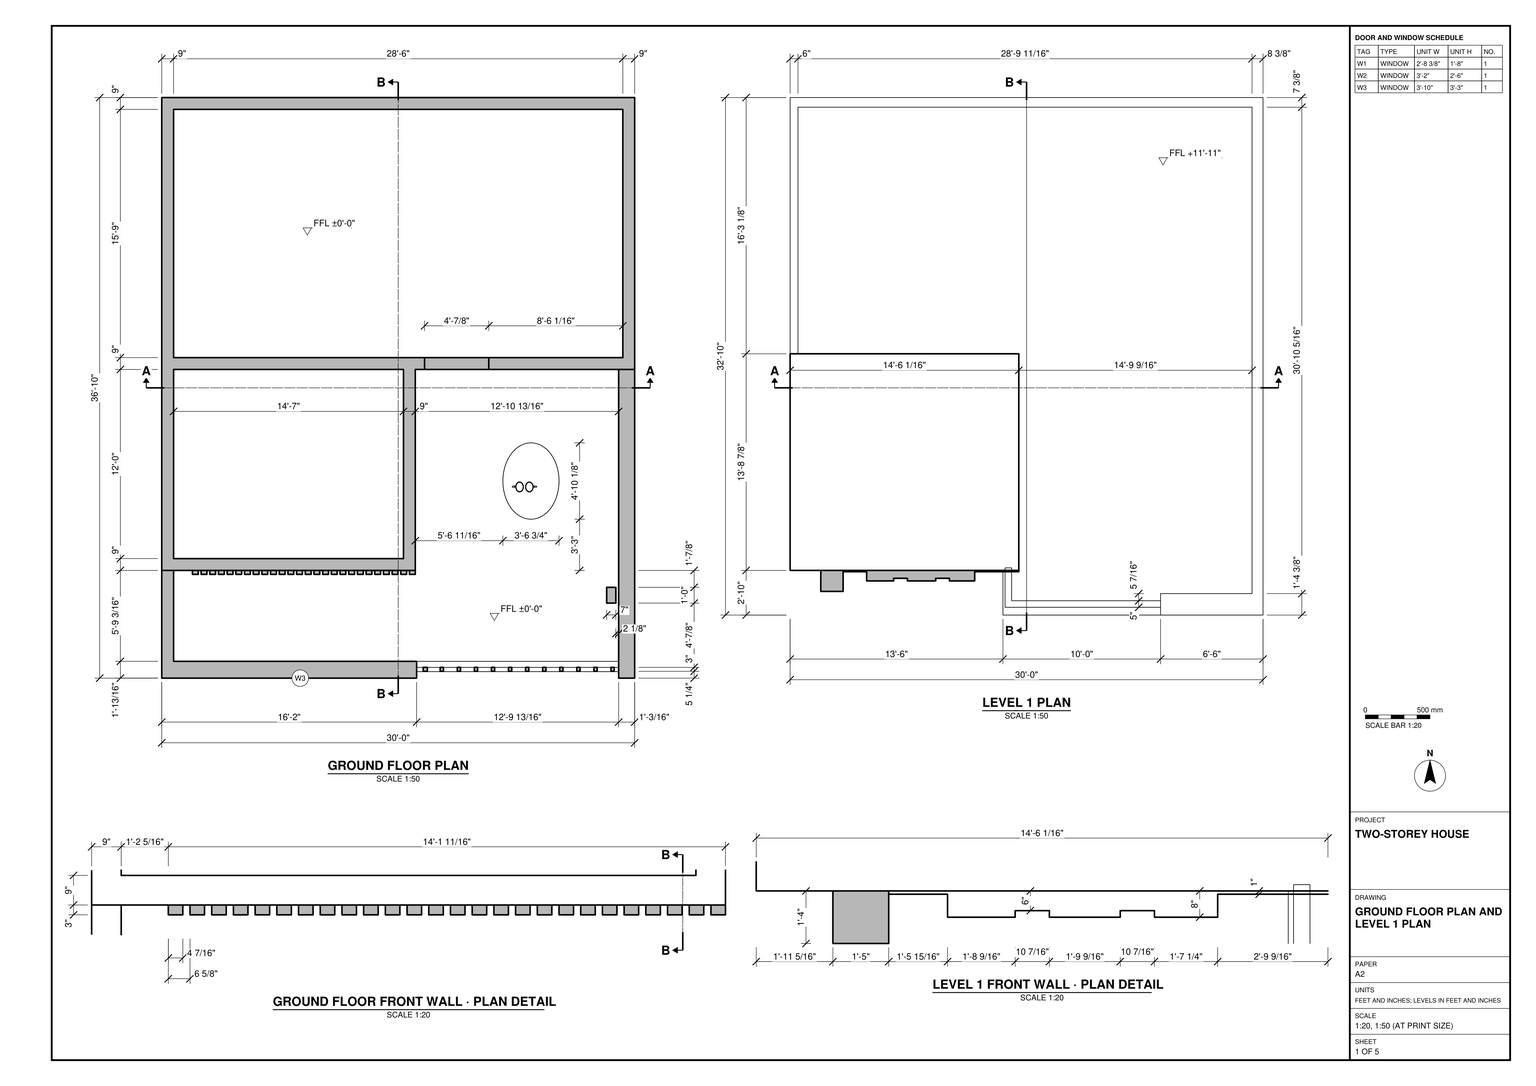
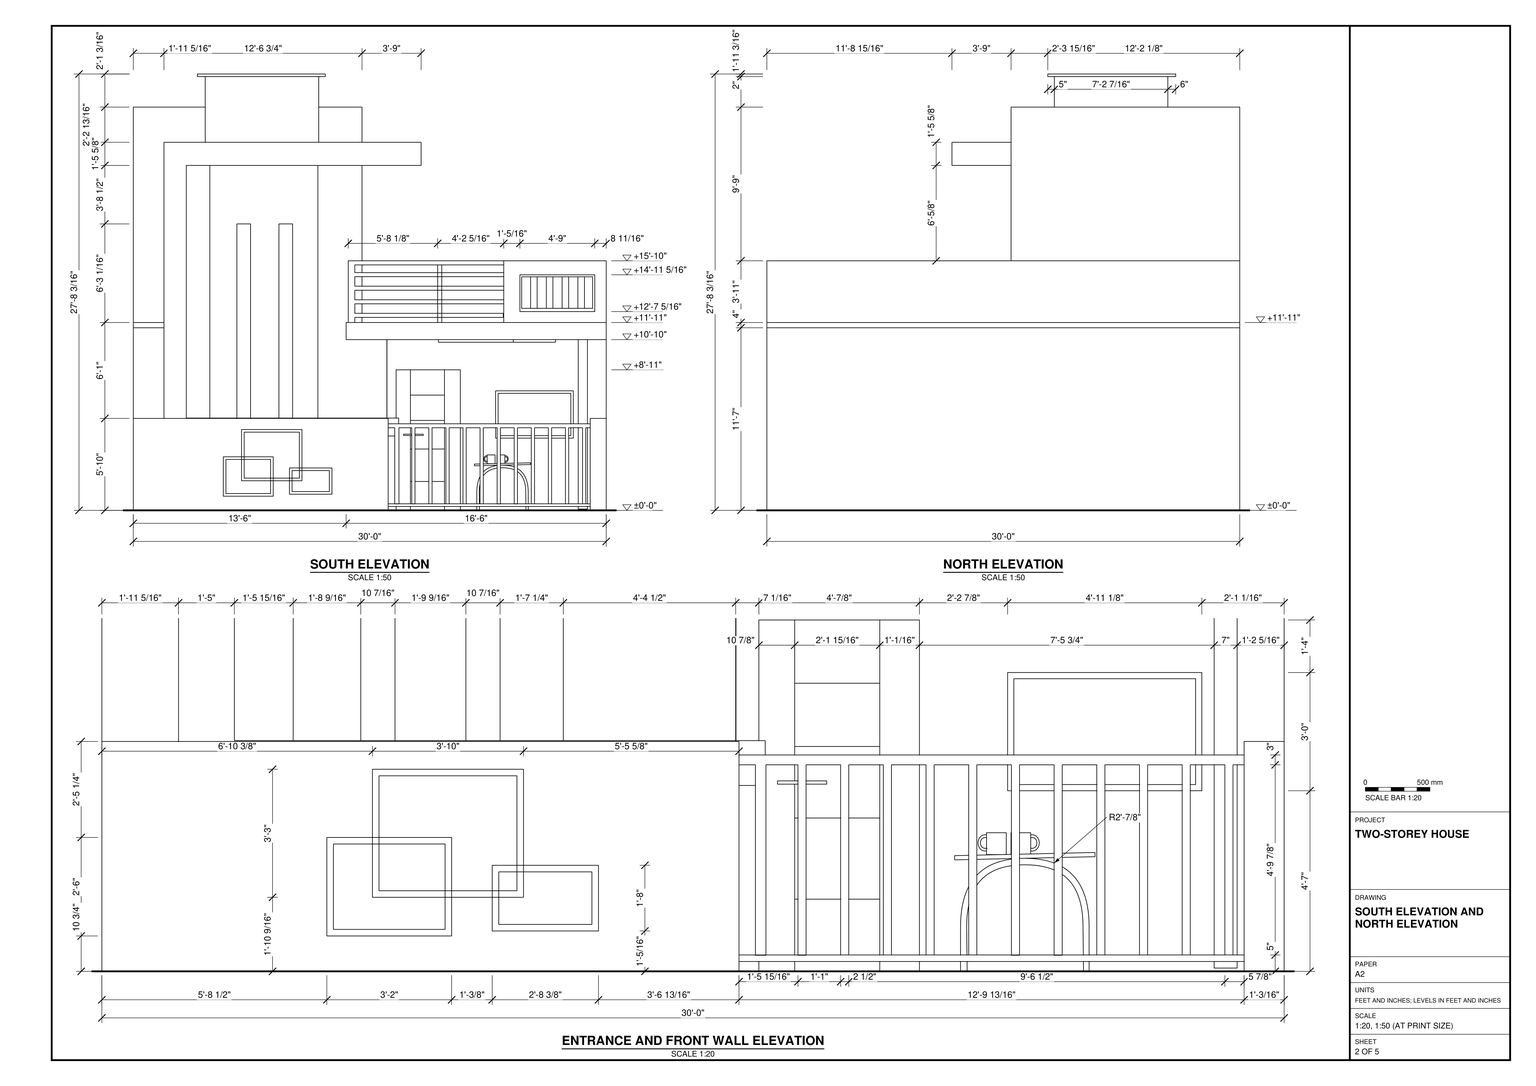
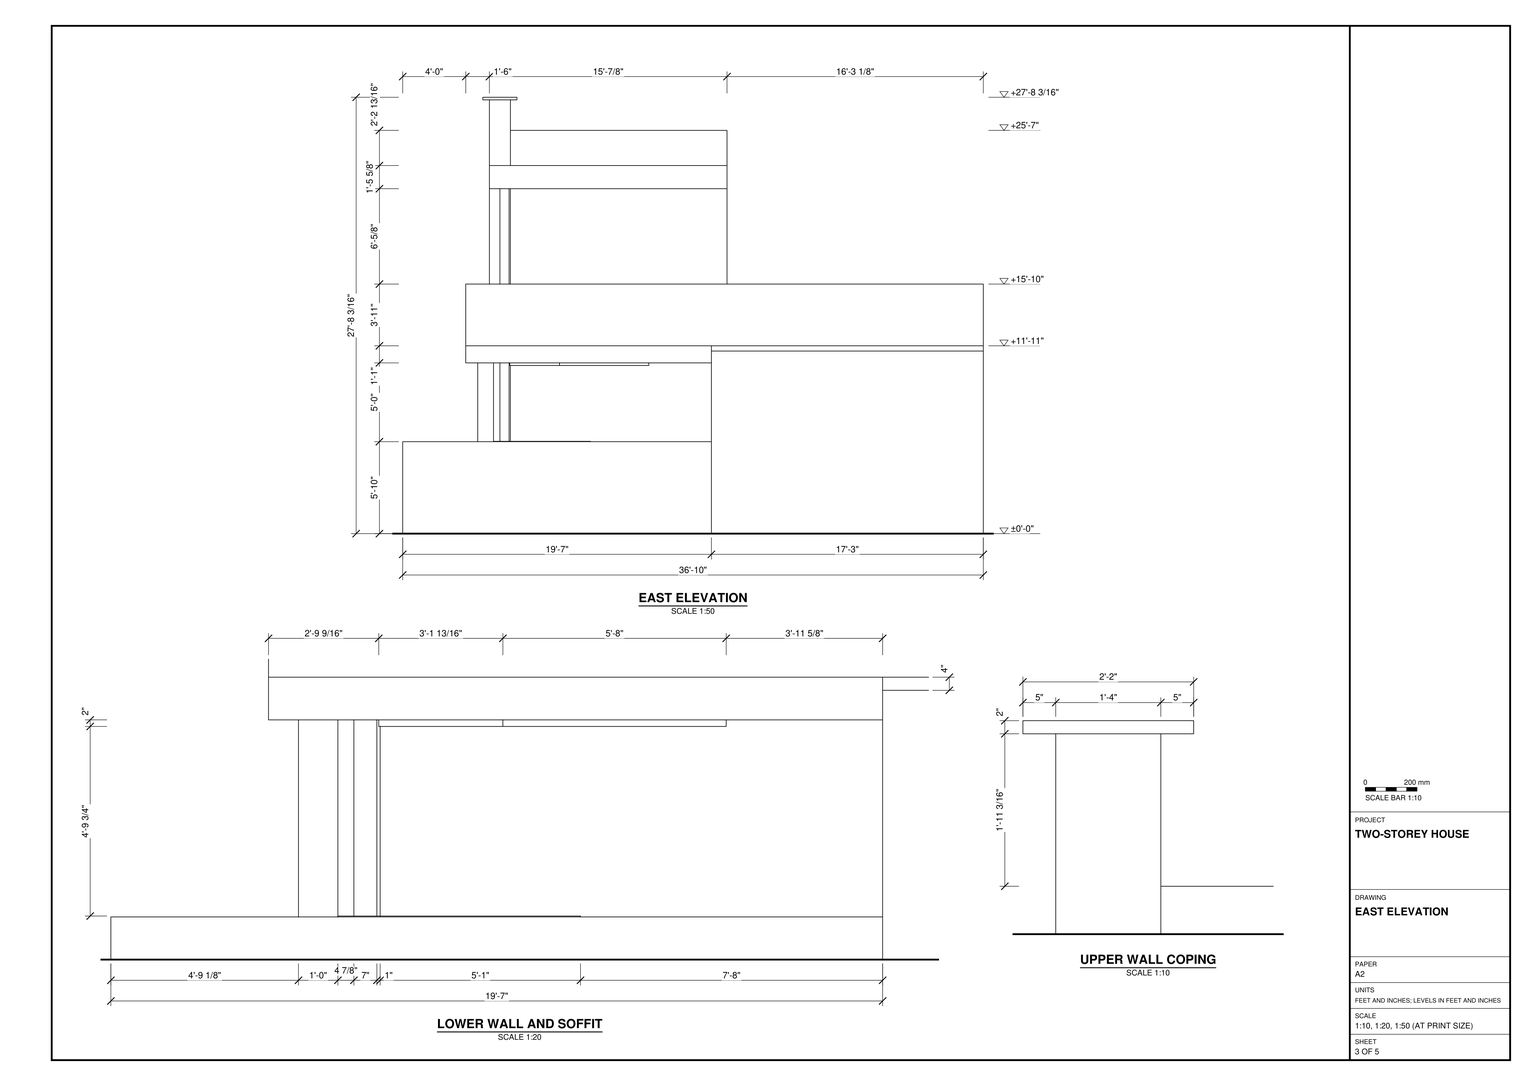
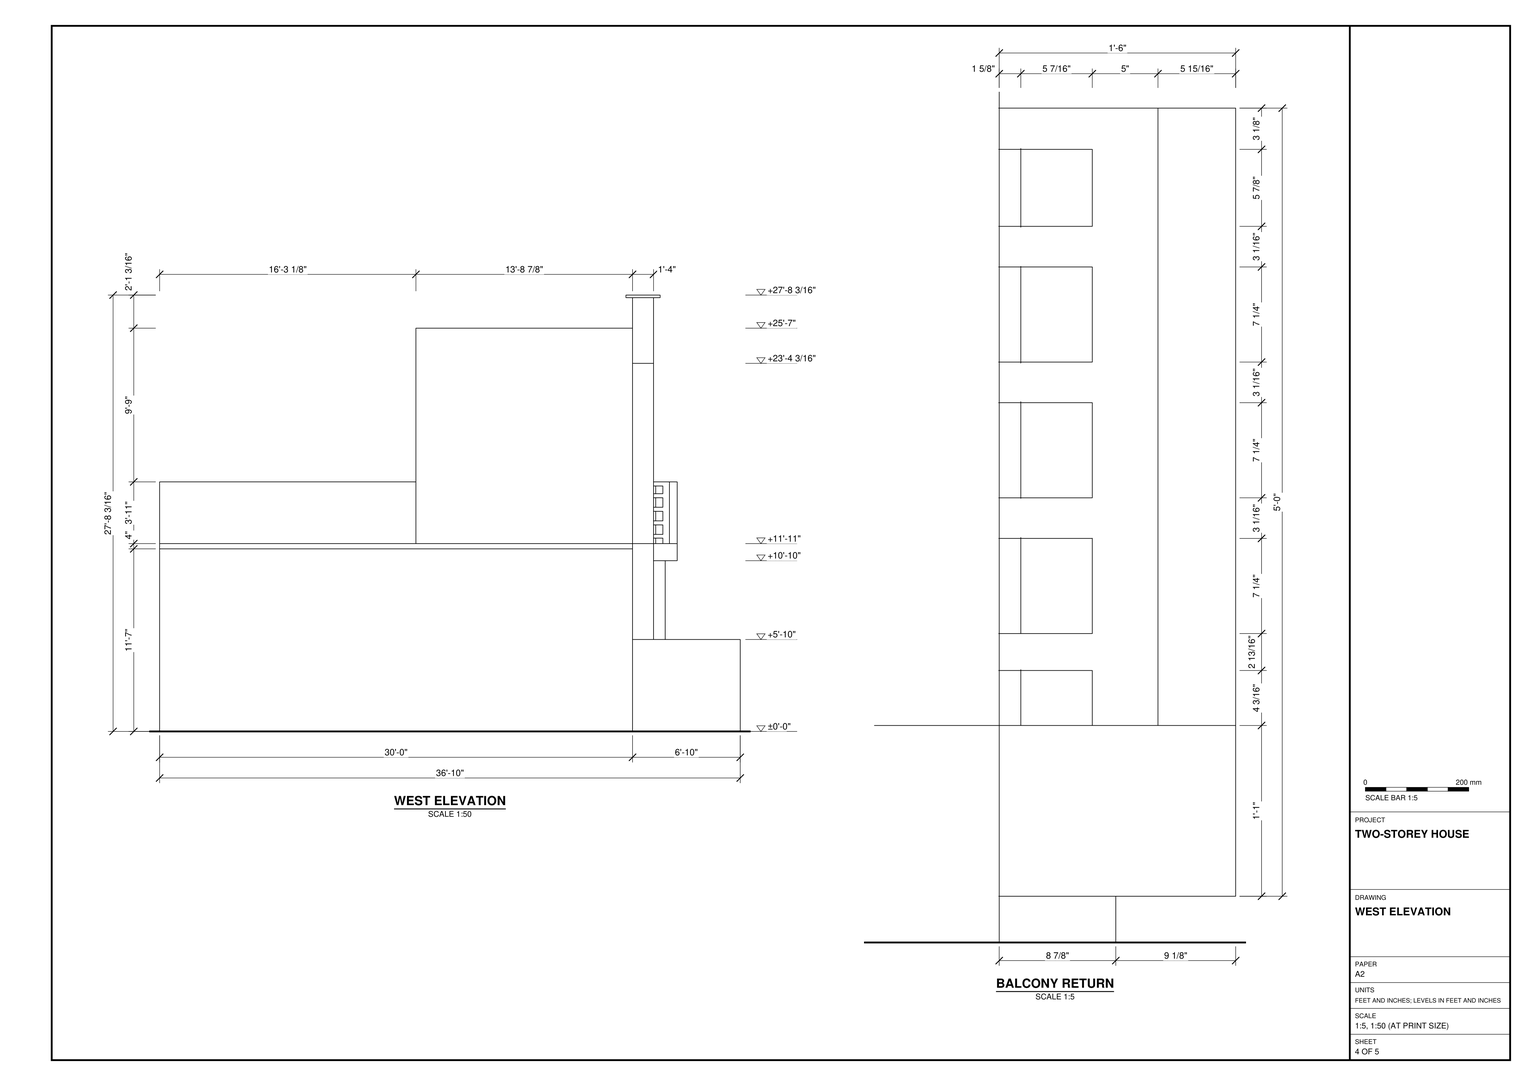
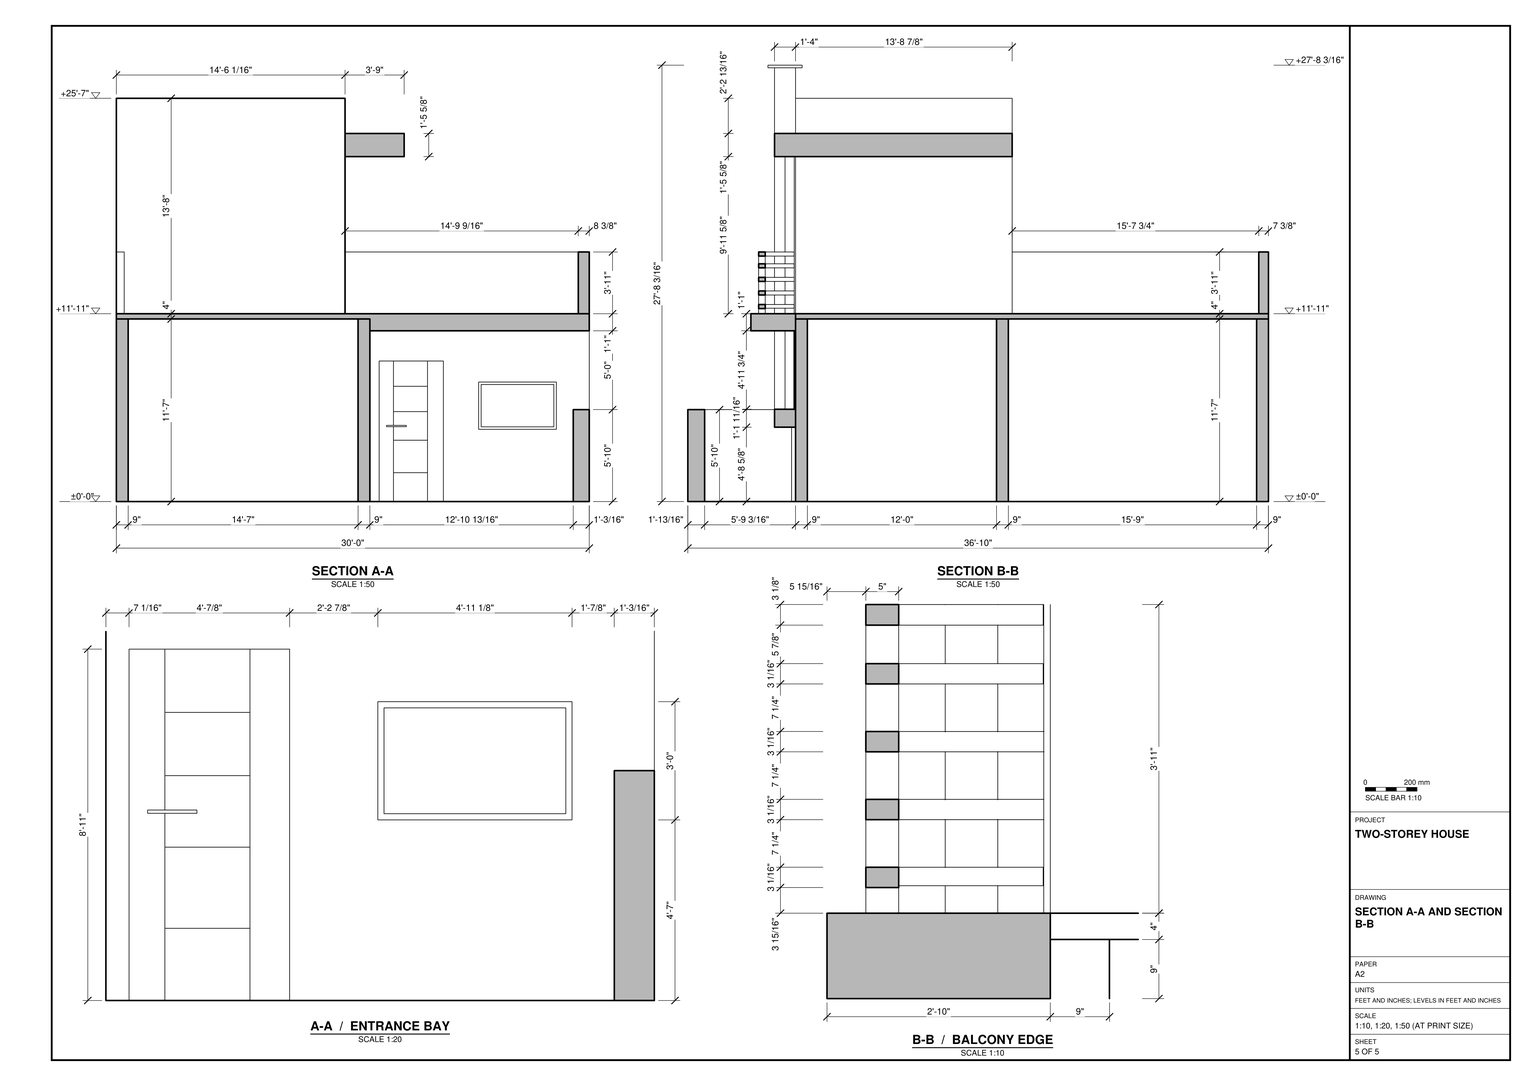
Build the two-storey house in SketchUp from task_files/diagram_01.pdf. Work in feet and inches. The house measures 30'-0" across the south frontage, 36'-10" from front to rear and 27'-8 3/16" high. Set the ground floor at ±0'-0" and level 1 at +11'-11".

Use the ground floor plan to lay out the full-width rear room, the smaller room to its front left and the open entrance area to the right. Follow the wall thicknesses shown, including the 9" walls around the rear room. On the south boundary, model the low wall with its three overlapping framed windows and the adjacent vertical-bar gate. Behind the gate, include the recessed entrance, its openings and the oval table in the position shown.

Build the floor and roof slabs, the set-back upper enclosure and the terrace to their drawn outlines. Use the south elevation to distinguish the tall projecting frame on the left from the lower terrace railing on the right. Follow the enlarged details for the front wall projections, slab soffit and upper wall coping. Decor and loose items may be any suitable library components.

Keep shell elements such as walls, slabs and roof in separate groups or components. Group each furniture or joinery piece separately and use components for repeated parts. Save one SketchUp model as output_files/two_storey_house_with_a_gated_forecourt_and_terrace.skp.

# SketchUp Ruby script. Lengths in inches.
U = 1.inch
M = Sketchup.active_model
def pt(a) = Geom::Point3d.new(a.map { |v| v * U })
def face(e, loops, mat)
  f = e.add_face(loops[0].map { |a| pt(a) })
  loops[1..].each { |l| e.add_face(l.map { |a| pt(a) }).erase! }
  f.material = f.back_material = mat if mat
  f
end
# faces: each face lists its corners as indices into pts; further lists are holes
def faces(e, pts, list, mat = nil) = list.each { |f| face(e, (f[0].is_a?(Array) ? f : [f]).map { |l| l.map { |i| pts[i] } }, mat) }
# xy, xz, yz: faces in a plane at the given z, y or x. An outline is a flat list of corners, or four numbers for a rectangle; further outlines are holes
def ring(l) = l.size == 4 ? [[l[0], l[1]], [l[2], l[1]], [l[2], l[3]], [l[0], l[3]]] : l.each_slice(2).to_a
def flat(e, list, mat, &to3) = list.each { |f| face(e, (f[0].is_a?(Array) ? f : [f]).map { |l| ring(l).map { |u, v| to3.(u, v) } }, mat) }
def xy(e, z, list, mat = nil) = flat(e, list, mat) { |x, y| [x, y, z] }
def xz(e, y, list, mat = nil) = flat(e, list, mat) { |x, z| [x, y, z] }
def yz(e, x, list, mat = nil) = flat(e, list, mat) { |y, z| [x, y, z] }
def lines(e, pts, list) = list.each { |a, b| e.add_line(pt(pts[a]), pt(pts[b])) }
# prism: a flat outline (further loops are holes) pulled along v
def prism(e, loops, v, mat = nil)
  f = face(e, loops, mat); d = Geom::Vector3d.new(v.map { |x| x * U })
  f.pushpull(f.normal.samedirection?(d) ? d.length : -d.length)
end
def box(e, o, s, mat = nil) = prism(e, [[o, [o[0] + s[0], o[1], o[2]], [o[0] + s[0], o[1] + s[1], o[2]], [o[0], o[1] + s[1], o[2]]]], [0, 0, s[2]], mat)
def at(x, y, z, deg = 0) = Geom::Transformation.translation(pt([x, y, z])) * Geom::Transformation.rotation(ORIGIN, Z_AXIS, deg.degrees)
def axes(o, x, y, z) = Geom::Transformation.new([*x, 0, *y, 0, *z, 0, *pt(o).to_a, 1])
def part(name) = M.definitions.add(name)
# library, detail: a bought-in or finely detailed component or shape, given as its bounding box
def library(name, o, s) = part(name).tap { |d| box(d.entities, o, s) }
def detail(e, o, s) = box(e.add_group.entities, o, s)
def put(e, d, t, mat = nil) = e.add_instance(d, t).tap { |i| i.material = mat if mat }
def group(e, t, mat = nil) = e.add_group.tap { |g| g.transformation = t; g.material = mat if mat }.entities
root = M.entities
M.materials.add("[Color A08]").color = [102, 0, 0]
M.materials.add("[Color C04]").color = [255, 153, 50]
M.materials.add("[Color C07]").color = [153, 76, 0]
M.materials.add("[Color M09]").color = [0, 0, 0]
M.materials.add("[Translucent Glass Blue]").color = [100, 149, 237]
M.materials["[Translucent Glass Blue]"].alpha = 0.5
c1 = part("Difference\#1")
xy(c1.entities,-19,[[[0,0,0,360,360,360,360,153,248.95,153,248.95,162,351,162,351,351,9,351,9,162,200.05,162,200.05,153,193,153,193,0],[9,9,184,153]]])
xy(c1.entities,36,[[275.81,153,334.94,162]])
xy(c1.entities,72,[[275.81,153,334.94,162]])
xy(c1.entities,88,[[200.05,153,248.95,162]])
xy(c1.entities,120,[[[0,0,193,0,193,153,360,153,360,360,0,360],[9,162,351,351],[9,9,184,153]]])
xz(c1.entities,0,[[0,-19,193,120]])
xz(c1.entities,9,[[9,-19,184,120]])
xz(c1.entities,153,[[9,-19,184,120],[[193,-19,200.05,-19,200.05,88,248.95,88,248.95,-19,360,-19,360,120,193,120],[275.81,36,334.94,72]]])
xz(c1.entities,162,[[[9,-19,9,120,351,120,351,-19,248.95,-19,248.95,88,200.05,88,200.05,-19],[275.81,36,334.94,72]]])
xz(c1.entities,351,[[9,-19,351,120]])
xz(c1.entities,360,[[0,-19,360,120]])
yz(c1.entities,0,[[0,-19,360,120]])
yz(c1.entities,9,[[9,-19,153,120],[162,-19,351,120]])
yz(c1.entities,184,[[9,-19,153,120]])
yz(c1.entities,193,[[0,-19,153,120]])
yz(c1.entities,200.05,[[153,-19,162,88]])
yz(c1.entities,248.95,[[153,-19,162,88]])
yz(c1.entities,275.81,[[153,36,162,72]])
yz(c1.entities,334.94,[[153,36,162,72]])
yz(c1.entities,351,[[162,-19,351,120]])
yz(c1.entities,360,[[153,-19,360,120]])
c2 = library("Group\#14",[0,0,0],[135.59,124.92,105.43])
xy(root,-19,[[0,0,0,82,9,82,9,12.78,194.01,12.78,194.01,0],[347.8125,0,360,235],[[9,12.78,347.8125,12.78,347.8125,235,360,235,360,442,0,442,0,82,9,82],[29.95,79,34.37,82],[49.78,79,54.2,82],[63,79,67.42,82],[23.34,79,27.76,82],[36.5625,79,40.98,82],[43.17,79,47.59,82],[56.39,79,60.8125,82],[69.61,79,74.03,82],[76.22,79,80.64,82],[82.83,79,87.25,82],[89.4375,79,93.86,82],[96.05,79,100.47,82],[102.66,79,107.08,82],[109.27,79,113.6875,82],[115.875,79,120.3,82],[122.48,79,126.91,82],[129.09,79,133.51,82],[135.7,79,140.125,82],[142.3125,79,146.73,82],[148.92,79,153.34,82],[155.53,79,159.95,82],[162.14,79,166.5625,82],[168.75,79,173.17,82],[175.36,79,179.78,82],[181.97,79,186.39,82],[188.58,79,193,82]],[23.34,79,27.76,82],[29.95,79,34.37,82],
  [36.5625,79,40.98,82],[43.17,79,47.59,82],[49.78,79,54.2,82],[56.39,79,60.8125,82],[63,79,67.42,82],
  [69.61,79,74.03,82],[76.22,79,80.64,82],[82.83,79,87.25,82],[89.4375,79,93.86,82],[96.05,79,100.47,82],
  [102.66,79,107.08,82],[109.27,79,113.6875,82],[115.875,79,120.3,82],[122.48,79,126.91,82],[129.09,79,133.51,82],
  [135.7,79,140.125,82],[142.3125,79,146.73,82],[148.92,79,153.34,82],[155.53,79,159.95,82],[162.14,79,166.5625,82],
  [168.75,79,173.17,82],[175.36,79,179.78,82],[181.97,79,186.39,82],[188.58,79,193,82]])
xy(root,-16,[[194.01,4.94,348.01,8.18]])
xy(root,-14.1,[[199.01,5.22,202.21,8.22],[211.96,5.22,214.43,8.22],[276.96,5.22,279.43,8.22],[289.96,5.22,292.43,8.22]])
xy(root,-14,[[224.96,5.22,227.43,8.18],[237.96,5.22,240.43,8.18],[250.96,5.22,253.43,8.18],[263.96,5.22,266.43,8.18],[302.96,5.22,305.43,8.18],
  [315.96,5.22,318.43,8.18],[328.96,5.22,331.43,8.18],[341.96,5.22,344.43,8.18],[224.96,8.18,227.43,8.22],[237.96,8.18,240.43,8.22],
  [250.96,8.18,253.43,8.22],[263.96,8.18,266.43,8.22],[302.96,8.18,305.43,8.22],[315.96,8.18,318.43,8.22],[328.96,8.18,331.43,8.22],
  [341.96,8.18,344.43,8.22]])
xy(root,-14,[[194.01,4.94,224.96,8.18],[224.96,4.94,227.43,5.22],[227.43,4.94,237.96,8.18],[237.96,4.94,240.43,5.22],[240.43,4.94,250.96,8.18],
  [250.96,4.94,253.43,5.22],[253.43,4.94,263.96,8.18],[263.96,4.94,266.43,5.22],[266.43,4.94,302.96,8.18],[302.96,4.94,305.43,5.22],
  [305.43,4.94,315.96,8.18],[315.96,4.94,318.43,5.22],[318.43,4.94,328.96,8.18],[328.96,4.94,331.43,5.22],[331.43,4.94,341.96,8.18],
  [341.96,4.94,344.43,5.22],[344.43,4.94,348.01,8.18]],"[Color M09]")
xy(root,37.61,[[23.34,79,27.76,82],[29.95,79,34.37,82],[36.5625,79,40.98,82],[43.17,79,47.59,82],[49.78,79,54.2,82],
  [56.39,79,60.8125,82],[63,79,67.42,82],[69.61,79,74.03,82],[76.22,79,80.64,82],[82.83,79,87.25,82],
  [89.4375,79,93.86,82],[96.05,79,100.47,82],[102.66,79,107.08,82],[109.27,79,113.6875,82],[115.875,79,120.3,82],
  [122.48,79,126.91,82],[129.09,79,133.51,82],[135.7,79,140.125,82],[142.3125,79,146.73,82],[148.92,79,153.34,82],
  [155.53,79,159.95,82],[162.14,79,166.5625,82],[168.75,79,173.17,82],[175.36,79,179.78,82],[181.97,79,186.39,82],
  [188.58,79,193,82]])
xy(root,43.9,[[194.01,5.22,199.01,8.22],[202.21,5.22,211.96,8.22],[214.43,5.22,224.96,8.22],[227.43,5.22,237.96,8.22],[240.43,5.22,250.96,8.22],
  [253.43,5.22,263.96,8.22],[266.43,5.22,276.96,8.22],[279.43,5.22,289.96,8.22],[292.43,5.22,302.96,8.22],[305.43,5.22,315.96,8.22],
  [318.43,5.22,328.96,8.22],[331.43,5.22,341.96,8.22],[344.43,5.22,349.01,8.22]])
xy(root,46.9,[[194.01,5.22,349.01,8.22]],"[Color M09]")
xy(root,51,[[0,0,194.01,0,194.01,12.78,9,12.78,9,82,0,82],[347.8125,0,360,235]])
xy(root,51.27,[[58.26,74,58.26,81,40.34,81,40.34,82,193.09,82,193.09,81,140.51,81,140.51,74,121.26,74,121.26,76,110.84,76,110.84,74,89.26,74,89.26,76,78.84,76,78.84,74]])
xy(root,111,[[174.09,81,193.09,82]])
xy(root,124,[[282,48,282,64.35,351.65,64.35,351.65,434.64,5.97,434.64,5.97,246.9,0,246.9,0,442,360,442,360,48],[163.62,53.91,168.62,58.91]])
xy(root,127.91,[[168.62,53.91,281.62,58.91]],"[Color M09]")
xy(root,128.1875,[[163.62,58.91,168.62,80.91]],"[Color M09]")
xy(root,131,[[168.62,53.91,281.62,58.91],[163.62,58.91,168.62,80.91]],"[Color M09]")
xy(root,134.82,[[[295.65,48,349.65,64.35],[302.41,53.61,307.41,57.61],[314.41,53.61,319.41,57.61],[326.41,53.61,331.41,57.61],[338.41,53.61,343.41,57.61]]])
xy(root,138.24,[[168.62,53.91,287.62,58.91],[163.62,58.91,168.62,83.91]],"[Color M09]")
xy(root,141.33,[[168.62,53.91,287.62,58.91],[163.62,58.91,168.62,83.91]],"[Color M09]")
xy(root,148.58,[[168.62,53.91,283.62,58.91],[163.62,58.91,168.62,81.91]],"[Color M09]")
xy(root,151.67,[[168.62,53.91,283.62,58.91],[163.62,58.91,168.62,81.91]],"[Color M09]")
xy(root,158.82,[[[295.65,48,349.65,64.35],[302.41,53.61,307.41,57.61],[314.41,53.61,319.41,57.61],[326.41,53.61,331.41,57.61],[338.41,53.61,343.41,57.61]]])
xy(root,158.91,[[168.62,53.91,285.62,58.91],[163.62,58.91,168.62,80.91]],"[Color M09]")
xy(root,162,[[168.62,53.91,285.62,58.91],[163.62,58.91,168.62,80.91]],"[Color M09]")
xy(root,167.86,[[168.62,53.91,231.71,58.91],[234.8,53.91,282,58.91],[163.62,58.91,168.62,80.91]],"[Color M09]")
xy(root,171,[[282,48,360,48,360,442,0,442,0,246.9,5.97,246.9,5.97,434.64,351.65,434.64,351.65,64.35,282,64.35]])
xy(root,171,[[163.62,53.91,282,53.91,282,58.91,168.62,58.91,168.62,80.91,163.62,80.91]],"[Color M09]")
xy(root,199.08,[[78.84,74,89.26,76],[110.84,74,121.26,76]])
xy(root,243.61,[[58.26,74,140.51,74,140.51,81,174.09,81,174.09,82,40.34,82,40.34,81,58.26,81]])
xy(root,261.22,[[54.74,66,141.14,82]])
xy(root,311.22,[[48.74,61,146.14,66],[48.74,66,54.74,82],[54.74,66,141.14,82],[141.14,66,146.14,82],[48.74,82,60.74,87],
  [60.74,82,146.14,87]])
xy(root,313.22,[[48.74,61,146.14,87]])
xz(root,0,[[0,-19,194.01,51],[347.8125,-19,360,51]])
xz(root,4.94,[[194.01,-16,348.01,-14]],"[Color M09]")
xz(root,5.22,[[199.01,-14.1,202.21,-14.1,202.21,43.9,211.96,43.9,211.96,-14.1,214.43,-14.1,214.43,43.9,224.96,43.9,224.96,-14,227.43,-14,227.43,43.9,237.96,43.9,237.96,-14,240.43,-14,240.43,43.9,250.96,43.9,250.96,-14,253.43,-14,253.43,43.9,263.96,43.9,263.96,-14,266.43,-14,266.43,43.9,276.96,43.9,276.96,-14.1,279.43,-14.1,279.43,43.9,289.96,43.9,289.96,-14.1,292.43,-14.1,292.43,43.9,302.96,43.9,302.96,-14,305.43,-14,305.43,43.9,315.96,43.9,315.96,-14,318.43,-14,318.43,43.9,328.96,43.9,328.96,-14,331.43,-14,331.43,43.9,341.96,43.9,341.96,-14,344.43,-14,344.43,43.9,349.01,43.9,349.01,46.9,194.01,46.9,194.01,43.9,199.01,43.9]],"[Color M09]")
xz(root,8.18,[[194.01,-16,348.01,-14]])
xz(root,8.22,[[199.01,-14.1,199.01,43.9,194.01,43.9,194.01,46.9,349.01,46.9,349.01,43.9,344.43,43.9,344.43,-14,341.96,-14,341.96,43.9,331.43,43.9,331.43,-14,328.96,-14,328.96,43.9,318.43,43.9,318.43,-14,315.96,-14,315.96,43.9,305.43,43.9,305.43,-14,302.96,-14,302.96,43.9,292.43,43.9,292.43,-14.1,289.96,-14.1,289.96,43.9,279.43,43.9,279.43,-14.1,276.96,-14.1,276.96,43.9,266.43,43.9,266.43,-14,263.96,-14,263.96,43.9,253.43,43.9,253.43,-14,250.96,-14,250.96,43.9,240.43,43.9,240.43,-14,237.96,-14,237.96,43.9,227.43,43.9,227.43,-14,224.96,-14,224.96,43.9,214.43,43.9,214.43,-14.1,211.96,-14.1,211.96,43.9,202.21,43.9,202.21,-14.1]])
xz(root,12.78,[[9,-19,194.01,51]])
xz(root,48,[[[282,124,360,171],[294.29,132.32,351.29,160.32]]])
xz(root,48,[[[294.29,132.32,351.29,160.32],[295.65,134.82,349.65,158.82]]],"[Color C07]")
xz(root,53.61,[[302.41,134.82,307.41,158.82],[314.41,134.82,319.41,158.82],[326.41,134.82,331.41,158.82],[338.41,134.82,343.41,158.82]])
xz(root,53.91,[[163.62,124,168.62,124,168.62,127.91,281.62,127.91,281.62,131,168.62,131,168.62,138.24,287.62,138.24,287.62,141.33,168.62,141.33,168.62,148.58,283.62,148.58,283.62,151.67,168.62,151.67,168.62,158.91,285.62,158.91,285.62,162,168.62,162,168.62,167.86,282,167.86,282,171,163.62,171]],"[Color M09]")
xz(root,57.61,[[302.41,134.82,307.41,158.82],[314.41,134.82,319.41,158.82],[326.41,134.82,331.41,158.82],[338.41,134.82,343.41,158.82]])
xz(root,58.91,[[163.62,124,163.62,128.1875,168.62,128.1875,168.62,131,281.62,131,281.62,127.91,168.62,127.91,168.62,124],[168.62,138.24,287.62,141.33],[168.62,148.58,283.62,151.67],[168.62,158.91,285.62,162],[168.62,167.86,282,171]])
xz(root,58.91,[[163.62,131,168.62,138.24],[163.62,141.33,168.62,148.58],[163.62,151.67,168.62,158.91],[163.62,162,168.62,167.86]],"[Color M09]")
xz(root,61,[[48.74,311.22,146.14,313.22]])
xz(root,64.35,[[[282,124,351.65,171],[295.65,134.82,349.65,158.82]]])
xz(root,66,[[54.74,261.22,141.14,311.22]])
xz(root,74,[[58.26,51.27,78.84,51.27,78.84,199.08,89.26,199.08,89.26,51.27,110.84,51.27,110.84,199.08,121.26,199.08,121.26,51.27,140.51,51.27,140.51,243.61,58.26,243.61]])
xz(root,76,[[78.84,51.27,89.26,199.08],[110.84,51.27,121.26,199.08]])
xz(root,79,[[23.34,-19,27.76,37.61],[29.95,-19,34.37,37.61],[36.5625,-19,40.98,37.61],[43.17,-19,47.59,37.61],[49.78,-19,54.2,37.61],
  [56.39,-19,60.8125,37.61],[63,-19,67.42,37.61],[69.61,-19,74.03,37.61],[76.22,-19,80.64,37.61],[82.83,-19,87.25,37.61],
  [89.4375,-19,93.86,37.61],[96.05,-19,100.47,37.61],[102.66,-19,107.08,37.61],[109.27,-19,113.6875,37.61],[115.875,-19,120.3,37.61],
  [122.48,-19,126.91,37.61],[129.09,-19,133.51,37.61],[135.7,-19,140.125,37.61],[142.3125,-19,146.73,37.61],[148.92,-19,153.34,37.61],
  [155.53,-19,159.95,37.61],[162.14,-19,166.5625,37.61],[168.75,-19,173.17,37.61],[175.36,-19,179.78,37.61],[181.97,-19,186.39,37.61],
  [188.58,-19,193,37.61]])
xz(root,80.91,[[163.62,128.1875,168.62,131],[163.62,158.91,168.62,162],[163.62,167.86,168.62,171]])
xz(root,81,[[40.34,51.27,58.26,243.61],[140.51,51.27,193.09,51.27,193.09,111,174.09,111,174.09,243.61,140.51,243.61]])
xz(root,81.91,[[163.62,148.58,168.62,151.67]])
xz(root,82,[[0,-19,9,51],[23.34,-19,27.76,37.61],[29.95,-19,34.37,37.61],[36.5625,-19,40.98,37.61],[43.17,-19,47.59,37.61],
  [49.78,-19,54.2,37.61],[56.39,-19,60.8125,37.61],[63,-19,67.42,37.61],[69.61,-19,74.03,37.61],[76.22,-19,80.64,37.61],
  [82.83,-19,87.25,37.61],[89.4375,-19,93.86,37.61],[96.05,-19,100.47,37.61],[102.66,-19,107.08,37.61],[109.27,-19,113.6875,37.61],
  [115.875,-19,120.3,37.61],[122.48,-19,126.91,37.61],[129.09,-19,133.51,37.61],[135.7,-19,140.125,37.61],[142.3125,-19,146.73,37.61],
  [148.92,-19,153.34,37.61],[155.53,-19,159.95,37.61],[162.14,-19,166.5625,37.61],[168.75,-19,173.17,37.61],[175.36,-19,179.78,37.61],
  [181.97,-19,186.39,37.61],[188.58,-19,193,37.61],[40.34,51.27,40.34,243.61,174.09,243.61,174.09,111,193.09,111,193.09,51.27],[54.74,261.22,141.14,311.22]])
xz(root,83.91,[[163.62,138.24,168.62,141.33]])
xz(root,87,[[48.74,311.22,146.14,313.22]])
xz(root,235,[[347.8125,-19,360,51]])
xz(root,235,[[[275.81,36,334.94,72],[277.69,37.89,333.05,70.11]]],"[Color A08]")
xz(root,235,[[277.69,37.89,333.05,70.11]],"[Translucent Glass Blue]")
xz(root,246.9,[[0,124,5.97,171]])
xz(root,434.64,[[5.97,124,351.65,171]])
xz(root,442,[[0,124,360,171]])
yz(root,0,[[0,-19,82,51],[246.9,124,442,171]])
yz(root,5.97,[[246.9,124,434.64,171]])
yz(root,9,[[12.78,-19,82,51]])
yz(root,23.34,[[79,-19,82,37.61]])
yz(root,27.76,[[79,-19,82,37.61]])
yz(root,29.95,[[79,-19,82,37.61]])
yz(root,34.37,[[79,-19,82,37.61]])
yz(root,36.5625,[[79,-19,82,37.61]])
yz(root,40.34,[[81,51.27,82,243.61]])
yz(root,40.98,[[79,-19,82,37.61]])
yz(root,43.17,[[79,-19,82,37.61]])
yz(root,47.59,[[79,-19,82,37.61]])
yz(root,48.74,[[61,311.22,87,313.22]])
yz(root,49.78,[[79,-19,82,37.61]])
yz(root,54.2,[[79,-19,82,37.61]])
yz(root,54.74,[[66,261.22,82,311.22]])
yz(root,56.39,[[79,-19,82,37.61]])
yz(root,58.26,[[74,51.27,81,243.61]])
yz(root,60.8125,[[79,-19,82,37.61]])
yz(root,63,[[79,-19,82,37.61]])
yz(root,67.42,[[79,-19,82,37.61]])
yz(root,69.61,[[79,-19,82,37.61]])
yz(root,74.03,[[79,-19,82,37.61]])
yz(root,76.22,[[79,-19,82,37.61]])
yz(root,78.84,[[74,51.27,76,199.08]])
yz(root,80.64,[[79,-19,82,37.61]])
yz(root,82.83,[[79,-19,82,37.61]])
yz(root,87.25,[[79,-19,82,37.61]])
yz(root,89.26,[[74,51.27,76,199.08]])
yz(root,89.4375,[[79,-19,82,37.61]])
yz(root,93.86,[[79,-19,82,37.61]])
yz(root,96.05,[[79,-19,82,37.61]])
yz(root,100.47,[[79,-19,82,37.61]])
yz(root,102.66,[[79,-19,82,37.61]])
yz(root,107.08,[[79,-19,82,37.61]])
yz(root,109.27,[[79,-19,82,37.61]])
yz(root,110.84,[[74,51.27,76,199.08]])
yz(root,113.6875,[[79,-19,82,37.61]])
yz(root,115.875,[[79,-19,82,37.61]])
yz(root,120.3,[[79,-19,82,37.61]])
yz(root,121.26,[[74,51.27,76,199.08]])
yz(root,122.48,[[79,-19,82,37.61]])
yz(root,126.91,[[79,-19,82,37.61]])
yz(root,129.09,[[79,-19,82,37.61]])
yz(root,133.51,[[79,-19,82,37.61]])
yz(root,135.7,[[79,-19,82,37.61]])
yz(root,140.125,[[79,-19,82,37.61]])
yz(root,140.51,[[74,51.27,81,243.61]])
yz(root,141.14,[[66,261.22,82,311.22]])
yz(root,142.3125,[[79,-19,82,37.61]])
yz(root,146.14,[[61,311.22,87,313.22]])
yz(root,146.73,[[79,-19,82,37.61]])
yz(root,148.92,[[79,-19,82,37.61]])
yz(root,153.34,[[79,-19,82,37.61]])
yz(root,155.53,[[79,-19,82,37.61]])
yz(root,159.95,[[79,-19,82,37.61]])
yz(root,162.14,[[79,-19,82,37.61]])
yz(root,163.62,[[53.91,124,53.91,171,80.91,171,80.91,167.86,58.91,167.86,58.91,162,80.91,162,80.91,158.91,58.91,158.91,58.91,151.67,81.91,151.67,81.91,148.58,58.91,148.58,58.91,141.33,83.91,141.33,83.91,138.24,58.91,138.24,58.91,131,80.91,131,80.91,128.1875,58.91,128.1875,58.91,124]],"[Color M09]")
yz(root,166.5625,[[79,-19,82,37.61]])
yz(root,168.62,[[53.91,124,58.91,127.91],[58.91,128.1875,80.91,131],[58.91,138.24,83.91,141.33],[58.91,148.58,81.91,151.67]])
yz(root,168.62,[[53.91,131,58.91,138.24],[53.91,141.33,58.91,148.58],[53.91,151.67,58.91,158.91],[58.91,158.91,80.91,162],[53.91,162,58.91,167.86],
  [58.91,167.86,80.91,171]],"[Color M09]")
yz(root,168.75,[[79,-19,82,37.61]])
yz(root,173.17,[[79,-19,82,37.61]])
yz(root,174.09,[[81,111,82,243.61]])
yz(root,175.36,[[79,-19,82,37.61]])
yz(root,179.78,[[79,-19,82,37.61]])
yz(root,181.97,[[79,-19,82,37.61]])
yz(root,186.39,[[79,-19,82,37.61]])
yz(root,188.58,[[79,-19,82,37.61]])
yz(root,193,[[79,-19,82,37.61]])
yz(root,193.09,[[81,51.27,82,111]])
yz(root,194.01,[[[0,-19,12.78,51],[5.22,43.9,8.22,46.9],[4.94,-16,8.18,-14]]])
yz(root,199.01,[[5.22,-14.1,8.22,43.9]])
yz(root,202.21,[[5.22,-14.1,8.22,43.9]],"[Color M09]")
yz(root,211.96,[[5.22,-14.1,8.22,43.9]])
yz(root,214.43,[[5.22,-14.1,8.22,43.9]],"[Color M09]")
yz(root,224.96,[[5.22,-14,8.22,43.9]])
yz(root,227.43,[[5.22,-14,8.22,43.9]],"[Color M09]")
yz(root,237.96,[[5.22,-14,8.22,43.9]])
yz(root,240.43,[[5.22,-14,8.22,43.9]],"[Color M09]")
yz(root,250.96,[[5.22,-14,8.22,43.9]])
yz(root,253.43,[[5.22,-14,8.22,43.9]],"[Color M09]")
yz(root,263.96,[[5.22,-14,8.22,43.9]])
yz(root,266.43,[[5.22,-14,8.22,43.9]],"[Color M09]")
yz(root,276.96,[[5.22,-14.1,8.22,43.9]])
yz(root,279.43,[[5.22,-14.1,8.22,43.9]],"[Color M09]")
yz(root,281.62,[[53.91,127.91,58.91,131]])
yz(root,282,[[48,124,48,171,53.91,171,53.91,167.86,58.91,167.86,58.91,171,64.35,171,64.35,124]])
yz(root,283.62,[[53.91,148.58,58.91,151.67]])
yz(root,285.62,[[53.91,158.91,58.91,162]])
yz(root,287.62,[[53.91,138.24,58.91,141.33]])
yz(root,289.96,[[5.22,-14.1,8.22,43.9]])
yz(root,292.43,[[5.22,-14.1,8.22,43.9]],"[Color M09]")
yz(root,295.65,[[48,134.82,64.35,158.82]])
yz(root,302.41,[[53.61,134.82,57.61,158.82]])
yz(root,302.96,[[5.22,-14,8.22,43.9]])
yz(root,305.43,[[5.22,-14,8.22,43.9]],"[Color M09]")
yz(root,307.41,[[53.61,134.82,57.61,158.82]])
yz(root,314.41,[[53.61,134.82,57.61,158.82]])
yz(root,315.96,[[5.22,-14,8.22,43.9]])
yz(root,318.43,[[5.22,-14,8.22,43.9]],"[Color M09]")
yz(root,319.41,[[53.61,134.82,57.61,158.82]])
yz(root,326.41,[[53.61,134.82,57.61,158.82]])
yz(root,328.96,[[5.22,-14,8.22,43.9]])
yz(root,331.41,[[53.61,134.82,57.61,158.82]])
yz(root,331.43,[[5.22,-14,8.22,43.9]],"[Color M09]")
yz(root,338.41,[[53.61,134.82,57.61,158.82]])
yz(root,341.96,[[5.22,-14,8.22,43.9]])
yz(root,343.41,[[53.61,134.82,57.61,158.82]])
yz(root,344.43,[[5.22,-14,8.22,43.9]],"[Color M09]")
yz(root,347.8125,[[0,-19,235,51]])
yz(root,348.01,[[4.94,-16,8.18,-14]])
yz(root,349.01,[[5.22,43.9,8.22,46.9]])
yz(root,349.65,[[48,134.82,64.35,158.82]])
yz(root,351.65,[[64.35,124,434.64,171]])
yz(root,360,[[0,-19,235,51],[48,124,442,171]])
p = [[263.39,185.36,109],[263.39,121.36,109],[319.39,121.36,109],[319.39,185.36,109]]
lines(root,p,[[0,1],[1,2],[2,3],[3,0]])
put(root,c1,at(0,82,0))
g1 = group(root,at(0,82,120))
xy(g1,-138,[[338.69,-24.875,345.69,-12.875]])
xy(g1,-9,[[[162,-34,162,0,193,0,193,153,360,153,360,-34],[338.69,-24.875,345.69,-12.875]]])
xy(g1,0,[[0,0,0,360,360,360,360,153,193,153,193,0]])
xy(g1,4,[[162,-34,360,-34,360,360,0,360,0,0,162,0]])
xz(g1,-34,[[162,-9,360,4]])
xz(g1,-24.875,[[338.69,-138,345.69,-9]])
xz(g1,-12.875,[[338.69,-138,345.69,-9]])
xz(g1,0,[[162,-9,193,0],[0,0,162,4],[162,0,193,4]])
xz(g1,153,[[193,-9,360,0]])
xz(g1,360,[[0,0,360,4]])
yz(g1,0,[[0,0,360,4]])
yz(g1,162,[[-34,-9,0,4]])
yz(g1,193,[[0,-9,153,0]])
yz(g1,338.69,[[-24.875,-138,-12.875,-9]])
yz(g1,345.69,[[-24.875,-138,-12.875,-9]])
yz(g1,360,[[-34,-9,153,4],[153,0,360,4]])
g2 = group(root,at(0,66,37.61))
xy(g2,0,[[23.34,0,23.34,16,193,16,193,77,202,77,202,0]])
xy(g2,13.66,[[40.34,0,202,0,202,77,193,77,193,16,40.34,16]])
xy(g2,86.39,[[0,16,174.09,180.9]])
xy(g2,206,[[40.34,0,40.34,16,174.09,16,174.09,180.9,219.09,180.9,219.09,0]])
xy(g2,223.61,[[23.34,0,219.09,0,219.09,180.9,174.09,180.9,174.09,16,23.34,16]])
xy(g2,250.39,[[0,16,174.09,180.9]])
xz(g2,0,[[23.34,0,202,0,202,13.66,40.34,13.66,40.34,206,219.09,206,219.09,223.61,23.34,223.61]])
xz(g2,16,[[23.34,0,23.34,86.39,40.34,86.39,40.34,13.66,193,13.66,193,0],[0,86.39,23.34,86.39,23.34,223.61,174.09,223.61,174.09,250.39,0,250.39],[23.34,86.39,40.34,86.39,40.34,206,174.09,206,174.09,223.61,23.34,223.61],[40.34,86.39,174.09,206]])
xz(g2,77,[[193,0,202,13.66]])
xz(g2,180.9,[[0,86.39,174.09,250.39],[174.09,206,219.09,223.61]])
yz(g2,0,[[16,86.39,180.9,250.39]])
yz(g2,23.34,[[0,0,16,86.39],[0,86.39,16,223.61]])
yz(g2,40.34,[[0,13.66,16,86.39],[0,86.39,16,206]])
yz(g2,174.09,[[16,86.39,180.9,206],[16,206,180.9,223.61],[16,223.61,180.9,250.39]])
yz(g2,193,[[16,0,77,13.66]])
yz(g2,202,[[0,0,77,13.66]])
yz(g2,219.09,[[0,206,180.9,223.61]])
g3 = group(root,at(200.05,233,-19))
xy(g3,0,[[0,2,48.9,11]],"[Color C07]")
xy(g3,57,[[5.66,0,20.66,2]],"[Color M09]")
xy(g3,58,[[5.66,0,20.66,2]],"[Color M09]")
xy(g3,107,[[0,2,48.9,11]],"[Color C07]")
xz(g3,0,[[5.66,57,20.66,58]],"[Color M09]")
xz(g3,2,[[10.91,0,36.82,21.99],[10.91,21.99,36.82,46.7],[10.91,46.7,36.82,46.7,36.82,68.48,10.91,68.48,10.91,58,20.66,58,20.66,57,10.91,57],[10.91,68.48,36.82,87.74],[10.91,87.74,36.82,107]],"[Color C04]")
xz(g3,2,[[0,0,10.91,0,10.91,57,5.66,57,5.66,58,10.91,58,10.91,107,0,107],[36.82,0,48.9,107]],"[Color C07]")
xz(g3,11,[[0,0,48.9,107]],"[Color C07]")
yz(g3,0,[[2,0,11,107]],"[Color C07]")
yz(g3,5.66,[[0,57,2,58]],"[Color M09]")
yz(g3,20.66,[[0,57,2,58]],"[Color M09]")
yz(g3,48.9,[[2,0,11,107]],"[Color C07]")
g4 = group(root,at(231.71,53.91,167.86),"[Color M09]")
box(g4,[0,0,-43.86],[3.09,5,43.86])
g5 = group(root,at(82.39,0,3.55))
xz(g5,0,[[[0,0,46,39],[2,2,44,37]]])
g6 = group(root,at(68.5,0,-8.22))
xz(g6,0,[[[0,0,38,30],[2,2,36,28]]])
g7 = group(root,at(118.86,0,-6.71))
xz(g7,0,[[[0,0,32.36,20],[2,2,30.36,18]]])
g8 = group(root,at(232.27,81.57,111))
xy(g8,-2,[[[0,0,57,64],[2,2,55,62]]])
xy(g8,0,[[[0,0,57,64],[2,2,55,62]],[2,2,55,62]])
xz(g8,0,[[0,-2,57,0]])
xz(g8,2,[[2,-2,55,0]])
xz(g8,62,[[2,-2,55,0]])
xz(g8,64,[[0,-2,57,0]])
yz(g8,0,[[0,-2,64,0]])
yz(g8,2,[[2,-2,62,0]])
yz(g8,55,[[2,-2,62,0]])
yz(g8,57,[[0,-2,64,0]])
g9 = group(root,at(261.39,119.36,111))
xy(g9,-2,[[[0,0,60,68],[2,2,58,66]]])
xy(g9,1,[[[0,0,60,68],[2,2,58,66]],[2,2,58,66]])
xz(g9,0,[[0,-2,60,1]])
xz(g9,68,[[0,-2,60,1]])
yz(g9,0,[[0,-2,68,1]])
yz(g9,60,[[0,-2,68,1]])
p = [[2,66,-2],[2,66,1],[58,66,-2],[58,66,1],[2,2,-2],[2,2,1],
  [58,2,-2],[58,2,1]]
lines(g9,p,[[0,1],[2,3],[4,5],[6,7]])
put(root,c2,axes([259.66,120.99,-19],[0.31544,0,0],[0,0.46546,0],[0,0,0.4004]))
